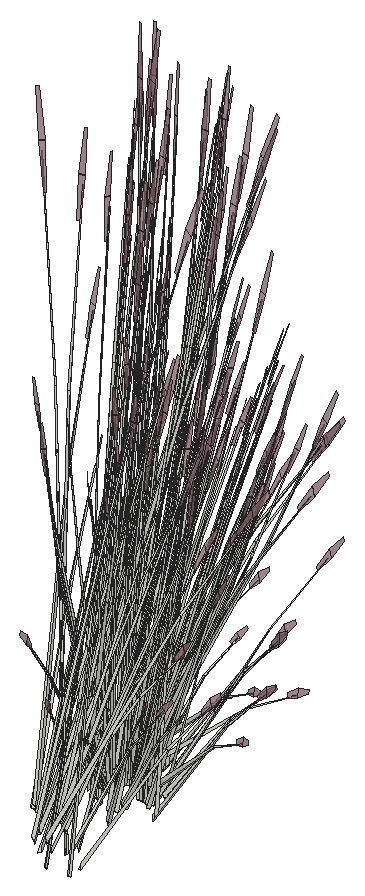
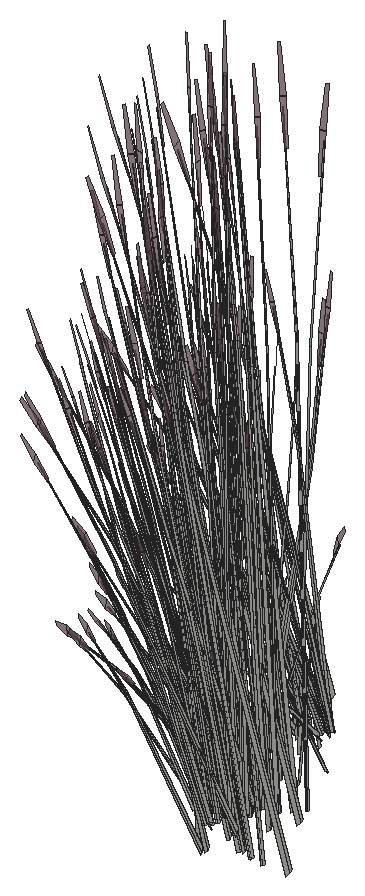
# SketchUp Ruby script. Lengths in inches.
U = 1.inch
M = Sketchup.active_model
def pt(a) = Geom::Point3d.new(a.map { |v| v * U })
def face(e, loops, mat)
  f = e.add_face(loops[0].map { |a| pt(a) })
  loops[1..].each { |l| e.add_face(l.map { |a| pt(a) }).erase! }
  f.material = f.back_material = mat if mat
  f
end
# faces: each face lists its corners as indices into pts; further lists are holes
def faces(e, pts, list, mat = nil) = list.each { |f| face(e, (f[0].is_a?(Array) ? f : [f]).map { |l| l.map { |i| pts[i] } }, mat) }
# xy, xz, yz: faces in a plane at the given z, y or x. An outline is a flat list of corners, or four numbers for a rectangle; further outlines are holes
def ring(l) = l.size == 4 ? [[l[0], l[1]], [l[2], l[1]], [l[2], l[3]], [l[0], l[3]]] : l.each_slice(2).to_a
def flat(e, list, mat, &to3) = list.each { |f| face(e, (f[0].is_a?(Array) ? f : [f]).map { |l| ring(l).map { |u, v| to3.(u, v) } }, mat) }
def xy(e, z, list, mat = nil) = flat(e, list, mat) { |x, y| [x, y, z] }
def xz(e, y, list, mat = nil) = flat(e, list, mat) { |x, z| [x, y, z] }
def yz(e, x, list, mat = nil) = flat(e, list, mat) { |y, z| [x, y, z] }
def lines(e, pts, list) = list.each { |a, b| e.add_line(pt(pts[a]), pt(pts[b])) }
# prism: a flat outline (further loops are holes) pulled along v
def prism(e, loops, v, mat = nil)
  f = face(e, loops, mat); d = Geom::Vector3d.new(v.map { |x| x * U })
  f.pushpull(f.normal.samedirection?(d) ? d.length : -d.length)
end
def box(e, o, s, mat = nil) = prism(e, [[o, [o[0] + s[0], o[1], o[2]], [o[0] + s[0], o[1] + s[1], o[2]], [o[0], o[1] + s[1], o[2]]]], [0, 0, s[2]], mat)
def at(x, y, z, deg = 0) = Geom::Transformation.translation(pt([x, y, z])) * Geom::Transformation.rotation(ORIGIN, Z_AXIS, deg.degrees)
def axes(o, x, y, z) = Geom::Transformation.new([*x, 0, *y, 0, *z, 0, *pt(o).to_a, 1])
def part(name) = M.definitions.add(name)
# library, detail: a bought-in or finely detailed component or shape, given as its bounding box
def library(name, o, s) = part(name).tap { |d| box(d.entities, o, s) }
def detail(e, o, s) = box(e.add_group.entities, o, s)
def put(e, d, t, mat = nil) = e.add_instance(d, t).tap { |i| i.material = mat if mat }
def group(e, t, mat = nil) = e.add_group.tap { |g| g.transformation = t; g.material = mat if mat }.entities
root = M.entities
M.materials.add("LightPink_Translucent").color = [144, 107, 117]
M.materials["LightPink_Translucent"].alpha = 0.75
c1 = part("blade")
p = [[2.15,0.21,22],[0,0.17,0],[0.09,0.45,0],[2.18,0.31,22],[2.29,0.31,22],[0.38,0.45,0],
  [2.48,0.24,33],[2.49,0.24,33],[2.48,0.22,33]]
faces(c1.entities,p,[[0,1,2,3],[4,5,2,3],[6,3,4,7],[8,0,3,6]])
c2 = part("seeds")
p = [[0.3,-0.1,1.38],[-0.01,-0.03,1.59],[-0.01,-0.03,0.03],[0.14,-0.07,-0.07],[0.29,-0.03,3],[0.15,0.01,3.11]]
faces(c2.entities,p,[[0,1,2,3],[1,0,4,5]],"LightPink_Translucent")
c3 = part("blade with seeds")
put(c3.entities,c1,at(0,0,0))
put(c3.entities,c2,axes([2.4,0.25,30.99],[1.5799,-0.05474,1.17369],[-0.12525,1.92788,0.29478],[-0.07173,-0.02425,1.56792]))
put(root,c3,axes([298.54,469.3,2.02],[0,0.65246,-0.49651],[-1.00089,0,0],[0,0.1486,1.57504]))
put(root,c3,axes([296.04,469.375,3.875],[-0.3323,-0.11241,1.71376],[0.68769,-0.4716,0.13857],[0.42861,0.21275,0.73262]))
put(root,c3,axes([295.54,477.44,4.72],[-0.00864,-0.12985,1.74944],[-0.72937,-0.3753,-0.27667],[0.11277,-0.2275,0.14031]))
put(root,c3,axes([296.1,467.9,4.47],[-0.77304,-0.33901,1.38283],[0.81626,-0.52782,0.59665],[0.24941,0.31809,1.33663]))
put(root,c3,axes([293.07,478.08,3.875],[-0.16657,0.22426,1.71376],[-0.69879,-0.4641,0.13857],[0.31524,-0.28926,0.73262]))
put(root,c3,axes([295.34,476.97,4.71],[-0.09085,0.04984,1.77383],[-0.89014,-0.16814,-0.16761],[-0.03222,-0.21748,0.31391]))
put(root,c3,axes([297.27,470.66,2.77],[-0.5037,-0.18761,1.1486],[0.6504,-0.19062,0.84392],[0.17543,0.16147,0.25299]))
put(root,c3,axes([295.5,471.19,5.03],[0.53309,-0.55848,-0.1216],[0.77201,0.32175,-0.67495],[0.26836,0.15779,1.02557]))
put(root,c3,axes([292.62,476.35,2.77],[0.11476,0.38047,1.1486],[-0.63664,-0.21072,0.84392],[0.06851,-0.19481,0.25299]))
put(root,c3,axes([293.97,478.18,4.68],[-0.64041,-0.4384,-0.51099],[0.67652,-0.38394,-0.3958],[0.09744,-0.22274,0.97773]))
put(root,c3,axes([296.52,471.13,2.375],[0.55932,0.6538,0],[-0.93577,0.36461,-0.51607],[-0.21313,0.08304,1.63711]))
put(root,c3,axes([294.8,471.65,4.71],[0.00265,-0.07899,1.77383],[0.76665,-0.34851,-0.16761],[0.2663,0.12439,0.31391]))
put(root,c3,axes([297.41,471.35,1.49],[0.06518,-0.0942,1.76342],[0.82057,-0.27742,-0.26939],[0.24877,0.14358,0.30037]))
put(root,c3,axes([296.33,469.21,2.09],[0.32803,0.59738,-0.69212],[-0.94492,0.21515,-0.18165],[0.03626,0.20229,1.52773]))
put(root,c3,axes([296.13,470.91,4.68],[0.88277,-0.1551,-0.51099],[0.15442,0.58737,-0.3958],[0.23711,0.16832,0.97773]))
put(root,c3,axes([293.68,471,5.05],[0.2697,-0.50175,0.35414],[0.78684,0.14635,-0.4572],[0.07215,0.20201,0.87481]))
put(root,c3,axes([294.65,478.41,5.03],[-0.98321,-0.03233,-0.1216],[0.02687,-0.61208,-0.67495],[0.0683,-0.23574,1.02557]))
put(root,c3,axes([294.58,478.02,4.53],[0.60531,-0.34352,-0.35414],[0.573,0.39225,0.4572],[0.08718,-0.19929,0.87481]))
put(root,c3,axes([297.35,471.51,2.67],[-0.57368,-0.02046,1.0506],[0.37886,-0.43461,0.58006],[0.22663,0.15441,0.8241]))
put(root,c3,axes([295.7,471.39,4.73],[-0.4066,0.41448,0.0643],[-0.57901,-0.24131,0.50621],[0.18719,0.13288,0.77189]))
put(root,c3,axes([294.74,472.79,5.65],[0.61821,-0.37431,-0.06488],[0.56645,0.40995,-0.29416],[0.03988,0.11616,0.97024]))
put(root,c3,axes([295.87,471.28,4.73],[-0.88979,0.14973,0.48003],[-0.15442,-0.58737,0.3958],[0.20926,0.17311,0.9933]))
put(root,c3,axes([295.48,470.46,2.59],[0.01579,-0.21629,1.43002],[0.75442,-0.24159,-0.30754],[0.23289,0.25887,0.61141]))
put(root,c3,axes([295.33,477.8125,1.49],[-0.1339,-0.0514,1.76342],[-0.34394,-0.57425,-0.26939],[0.23202,-0.15583,0.30037]))
put(root,c3,axes([293.44,471.46,4.73],[-0.6592,0.22175,0.0643],[-0.32265,-0.40436,0.50621],[0.06366,0.17825,0.77189]))
put(root,c3,axes([293.42,471.21,5.03],[0.87543,-0.30377,-0.1216],[0.4302,0.53915,-0.67495],[0.1155,0.2272,1.02557]))
put(root,c3,axes([293.67,471.41,5.0625],[-0.88151,-0.17057,0.53283],[0.30143,-0.56078,0.43934],[0.05297,0.22053,1.10256]))
put(root,c3,axes([294.57,478.15,4.73],[0.63704,0.44518,0.48003],[-0.67652,0.38394,0.3958],[0.11751,-0.20886,0.9933]))
put(root,c3,axes([294.81,478.2,4.73],[0.73517,0.0304,0.0643],[-0.02016,0.45906,0.50621],[0.07693,-0.17585,0.77189]))
put(root,c3,axes([293.58,471.33,1.49],[0.14478,-0.0355,1.76342],[0.8709,0.19542,-0.26939],[0.02547,0.22025,0.30037]))
put(root,c3,axes([294.26,478.51,5.05],[-0.60531,0.34352,0.35414],[-0.573,-0.39225,-0.4572],[0.08718,-0.19929,0.87481]))
put(root,c3,axes([295.33,479.43,4.98],[0.4673,-0.51481,-0.71045],[0.81887,0.36587,0.08574],[0.27902,-0.18652,1.00501]))
put(root,c3,axes([290.28,477.93,2.375],[-0.55932,-0.6538,0],[0.93577,-0.36461,-0.51607],[0.21313,-0.08304,1.63711]))
put(root,c3,axes([295.3,479.19,4.68],[-0.22982,-0.59576,-0.51099],[0.87033,-0.10422,-0.3958],[0.24941,-0.16002,0.97773]))
put(root,c3,axes([294.17,471.1875,4.68],[0.87941,0.16356,-0.51099],[-0.30143,0.56078,-0.3958],[0.08064,0.22578,0.97773]))
put(root,c3,axes([294.67,470.03,3.875],[-0.2045,-0.20949,1.71376],[0.94495,-0.17636,0.13857],[0.21357,0.32887,0.73262]))
put(root,c3,axes([295.72,479.62,5.03],[-0.82753,-0.35977,-0.1216],[0.47675,-0.52101,-0.67495],[0.2338,-0.18111,1.02557]))
put(root,c3,axes([293.77,471.53,4.53],[-0.2697,0.50175,-0.35414],[-0.78684,-0.14635,0.4572],[0.07215,0.20201,0.87481]))
put(root,c3,axes([291.04,477.83,2.02],[0.83726,-0.32623,-0.49651],[0.50045,0.58498,0],[0.19069,-0.0743,1.57504]))
put(root,c3,axes([296,478.96,2.59],[-0.31959,-0.01933,1.43002],[-0.32741,-0.51843,-0.30754],[0.39262,-0.14666,0.61141]))
put(root,c3,axes([297.75,479.46,4.71],[-0.11685,-0.00496,1.77383],[-0.48522,-0.53096,-0.16761],[0.19486,-0.17458,0.31391]))
put(root,c3,axes([292.03,479.17,2.06],[0.60257,-0.49041,-0.62353],[0.74854,0.44469,-0.16365],[0.24146,-0.12234,1.37633]))
put(root,c3,axes([296.37,478.01,2.77],[-0.29798,0.33213,1.1486],[-0.25612,-0.44624,0.84392],[0.24611,-0.11182,0.25299]))
put(root,c3,axes([293.85,471.08,4.98],[0.42698,0.53052,-0.71045],[-0.87893,0.29566,0.08574],[0.09984,0.25633,1.00501]))
put(root,c3,axes([295.95,479.25,4.53],[0.77872,-0.09325,-0.35414],[0.20563,0.53305,0.4572],[0.22316,-0.14318,0.87481]))
put(root,c3,axes([293.21,472.42,4.72],[0.1134,0.10507,1.74944],[0.91515,0.04128,-0.27667],[0.09203,0.23172,0.14031]))
put(root,c3,axes([291.375,479.74,2.67],[-0.10425,-0.7445,-0.29095],[1.08575,-0.04502,-0.50002],[0.19119,-0.09917,1.59708]))
put(root,c3,axes([295.3125,479.57,5.05],[-0.77872,0.09325,0.35414],[-0.20563,-0.53305,-0.4572],[0.22316,-0.14318,0.87481]))
put(root,c3,axes([291.23,478.09,2.03],[0.83462,0.16144,-0.30978],[-0.21015,0.56852,0.30978],[0.16826,-0.06556,1.38974]))
put(root,c3,axes([296.02,479.48,4.73],[0.61415,0.2744,0.0643],[-0.35756,0.39076,0.50621],[0.1969,-0.12633,0.77189]))
put(root,c3,axes([295.85,479.37,4.73],[0.22187,0.60049,0.48003],[-0.87033,0.10422,0.3958],[0.25651,-0.14123,0.9933]))
put(root,c3,axes([298.19,480.1,4.72],[0.12414,-0.09938,1.74944],[-0.15889,-0.60963,-0.27667],[0.31148,-0.11559,0.14031]))
put(root,c3,axes([295.75,481.02,5.03],[-0.45012,-0.59081,-0.1216],[0.79888,-0.29033,-0.67495],[0.33665,-0.07795,1.02557]))
put(root,c3,axes([295.71,480.51,4.68],[0.24236,-0.59349,-0.51099],[0.83094,0.20343,-0.3958],[0.33455,-0.05442,0.97773]))
put(root,c3,axes([294.4,478.1,2.375],[0.55932,-0.6538,0],[0.93577,0.36461,-0.51607],[0.21313,0.08304,1.63711]))
put(root,c3,axes([296.6,480.68,1.98],[-0.57619,0.0783,1.41583],[-0.09171,-0.62326,0.08104],[0.40356,-0.09434,0.80566]))
put(root,c3,axes([297.65,480.13,2.26],[-0.55463,-0.41721,-0.06488],[0.60744,-0.38228,-0.29416],[0.17212,-0.02691,0.97024]))
put(root,c3,axes([293.91,478.4375,2.48],[-0.83726,-0.32623,0.49651],[0.50045,-0.58498,0],[0.19069,0.0743,1.57504]))
put(root,c3,axes([295.55,480.73,4.98],[0.78611,-0.28816,-0.71045],[0.4381,0.59317,0.08574],[0.37982,-0.06738,1.00501]))
put(root,c3,axes([291.55,483.7,4.72],[-0.00864,-0.12985,1.74944],[-0.72937,-0.3753,-0.27667],[0.11277,-0.2275,0.14031]))
put(root,c3,axes([289.08,484.34,3.875],[-0.16657,0.22426,1.71376],[-0.69879,-0.4641,0.13857],[0.31524,-0.28926,0.73262]))
put(root,c3,axes([292.03,479.71,2.36],[-0.74176,0.59212,0.45755],[-0.88124,-0.52269,0.17955],[0.17882,-0.05909,1.58856]))
put(root,c3,axes([295.44,480.84,5.05],[-0.74348,-0.18202,0.35414],[0.21685,-0.53102,-0.4572],[0.29933,-0.04869,0.87481]))
put(root,c3,axes([290.35,479.26,1.59],[-0.88056,0.26122,1.28929],[-0.28027,-0.74951,0.50096],[0.54072,0.01247,1.46642]))
put(root,c3,axes([292.71,479.45,2.62],[0.17258,-0.58229,0.1448],[0.84319,0.10108,-0.41347],[0.15345,0.05979,1.26744]))
put(root,c3,axes([297.23,480.27,1.49],[-0.04675,-0.09906,1.76342],[0.32428,-0.57943,-0.26939],[0.32711,-0.00833,0.30037]))
put(root,c3,axes([292.35,479.61,2.72],[-0.53742,-0.54764,0.44739],[0.81403,-0.38564,-0.21531],[0.17391,0.06776,1.43643]))
put(root,c3,axes([292.63,479.64,2.67],[0.90324,-0.43318,-0.29095],[0.60064,0.61207,-0.50002],[0.22285,0.06216,1.59708]))
put(root,c3,axes([296.22,480.79,4.53],[0.74348,0.18202,-0.35414],[-0.21685,0.53102,0.4572],[0.29933,-0.04869,0.87481]))
put(root,c3,axes([294.9,478.49,2.02],[0.83726,0.32623,-0.49651],[-0.50045,0.58498,0],[0.19069,0.0743,1.57504]))
put(root,c3,axes([293.32,480.35,2.21],[1.00089,0,0],[0,0.67548,0],[0,0,1.78407]))
put(root,c3,axes([293.6,478.77,2.47],[-0.96132,0.17317,0.17642],[-0.23737,-0.64447,0.35086],[0.08574,0.0939,1.60407]))
put(root,c3,axes([294.19,480.13,3.875],[-0.37107,0.01478,1.71376],[0.24616,-0.64047,0.13857],[0.5288,0.03961,0.73262]))
put(root,c3,axes([294.67,478.73,2.03],[0.21015,0.56852,-0.30978],[-0.83462,0.16144,0.30978],[0.16826,0.06556,1.38974]))
put(root,c3,axes([296.11,481.01,4.73],[0.32857,0.44488,0.0643],[-0.59916,0.21775,0.50621],[0.26412,-0.04296,0.77189]))
put(root,c3,axes([292.99,480.01,2.38],[-1.13071,-0.13747,0.49198],[0.23011,-0.77639,0.19306],[0.16524,0.07497,1.70813]))
put(root,c3,axes([296.05,480.85,4.73],[-0.25275,0.59491,0.48003],[-0.83094,-0.20343,0.3958],[0.32677,-0.03575,0.9933]))
put(root,c3,axes([291.35,484.07,1.49],[-0.1339,-0.0514,1.76342],[-0.34394,-0.57425,-0.26939],[0.23202,-0.15583,0.30037]))
put(root,c3,axes([293.18,481.85,2.18],[0.93921,-0.22138,-0.19198],[0.33003,0.6377,0.00008],[0.10367,-0.02447,1.73897]))
put(root,c3,axes([293.29,480.64,2.21],[0.62448,0.42144,0],[-0.62448,0.42144,0],[0,0,1.69266]))
put(root,c3,axes([290.59,484.41,4.73],[0.63704,0.44518,0.48003],[-0.67652,0.38394,0.3958],[0.11751,-0.20886,0.9933]))
put(root,c3,axes([290.82,484.46,4.73],[0.73517,0.0304,0.0643],[-0.02016,0.45906,0.50621],[0.07693,-0.17585,0.77189]))
put(root,c3,axes([293.68,479.74,2.06],[0.9306,0.10697,-0.62353],[-0.19638,0.65984,-0.16365],[0.27771,0.07995,1.37633]))
put(root,c3,axes([297.8,480.89,2.77],[-0.55274,0.10771,1.1486],[0.26018,-0.44517,0.84392],[0.29323,0.03046,0.25299]))
put(root,c3,axes([291.34,485.69,4.98],[0.4673,-0.51481,-0.71045],[0.81887,0.36587,0.08574],[0.27902,-0.18652,1.00501]))
put(root,c3,axes([291.32,485.45,4.68],[-0.22982,-0.59576,-0.51099],[0.87033,-0.10422,-0.3958],[0.24941,-0.16002,0.97773]))
put(root,c3,axes([293.29,480.15,2.72],[0.43405,-0.58792,0.44739],[0.90188,0.28295,-0.21531],[0,0.13553,1.43643]))
put(root,c3,axes([297.54,482.78,4.71],[-0.08089,-0.05712,1.77383],[0.17695,-0.61228,-0.16761],[0.31864,-0.03912,0.31391]))
put(root,c3,axes([291.73,485.88,5.03],[-0.82753,-0.35977,-0.1216],[0.47675,-0.52101,-0.67495],[0.2338,-0.18111,1.02557]))
put(root,c3,axes([293.2,479.95,2.21],[0.53742,0.54764,-0.44739],[-0.81403,0.38564,0.21531],[0.17391,0.06776,1.43643]))
put(root,c3,axes([296.84,482.27,3.93],[-0.17122,-0.54847,-0.03492],[0.80929,-0.12609,-0.15832],[0.169,0.03477,0.52218]))
put(root,c3,axes([294.74,482.25,5.03],[0.0479,-0.66354,-0.1216],[0.90696,0.01814,-0.67495],[0.3493,0.04609,1.02557]))
put(root,c3,axes([295.5625,480.48,2.48],[0,-0.65246,0.49651],[1.00089,0,0],[0,0.1486,1.57504]))
put(root,c3,axes([293.66,480.28,2.62],[0.83351,-0.19028,0.1448],[0.29189,0.54335,-0.41347],[0,0.11958,1.26744]))
put(root,c3,axes([294.6,481.99,5.05],[-0.50902,-0.40851,0.35414],[0.58122,-0.38671,-0.4572],[0.29531,0.05884,0.87481]))
put(root,c3,axes([292.02,485.22,2.59],[-0.31959,-0.01933,1.43002],[-0.32741,-0.51843,-0.30754],[0.39262,-0.14666,0.61141]))
put(root,c3,axes([293.77,485.72,4.71],[-0.11685,-0.00496,1.77383],[-0.48522,-0.53096,-0.16761],[0.19486,-0.17458,0.31391]))
put(root,c3,axes([296.76,481.61,2.59],[-0.21545,-0.16047,1.43002],[0.28033,-0.53085,-0.30754],[0.43591,0.07191,0.61141]))
put(root,c3,axes([288.04,485.43,2.06],[0.60257,-0.49041,-0.62353],[0.74854,0.44469,-0.16365],[0.24146,-0.12234,1.37633]))
put(root,c3,axes([292.39,484.27,2.77],[-0.29798,0.33213,1.1486],[-0.25612,-0.44624,0.84392],[0.24611,-0.11182,0.25299]))
put(root,c3,axes([292.91,482.19,2.2],[0.90188,0.29293,0],[-0.43405,0.60866,0],[0,0,1.74954]))
put(root,c3,axes([291.96,485.51,4.53],[0.77872,-0.09325,-0.35414],[0.20563,0.53305,0.4572],[0.22316,-0.14318,0.87481]))
put(root,c3,axes([295.53,481.85,4.72],[0.19191,-0.01103,1.74944],[0.52639,-0.5069,-0.27667],[0.34136,0.06691,0.14031]))
put(root,c3,axes([291.33,485.83,5.05],[-0.77872,0.09325,0.35414],[-0.20563,-0.53305,-0.4572],[0.22316,-0.14318,0.87481]))
put(root,c3,axes([294.78,481.93,4.98],[0.89428,0.01571,-0.71045],[-0.06006,0.66153,0.08574],[0.37886,0.06981,1.00501]))
put(root,c3,axes([296.24,480.59,2.375],[1.11865,0,0],[0,0.72922,-0.51607],[0,0.16609,1.63711]))
put(root,c3,axes([295.8,480.96,2.2],[-1.1181,-0.00522,-0.04976],[0,-0.72922,0.49943],[-0.03514,0.166,1.58352]))
put(root,c3,axes([293.375,480.33,2.67],[1.00749,0.31132,-0.29095],[-0.48511,0.65709,-0.50002],[0.03166,0.16133,1.59708]))
put(root,c3,axes([292.03,485.75,4.73],[0.61415,0.2744,0.0643],[-0.35756,0.39076,0.50621],[0.1969,-0.12633,0.77189]))
put(root,c3,axes([295.32,482.2,4.53],[0.50902,0.40851,-0.35414],[-0.58122,0.38671,0.4572],[0.29531,0.05884,0.87481]))
put(root,c3,axes([295.5625,481.07,2.03],[-0.62448,0.40708,-0.30978],[-0.62448,-0.40708,0.30978],[0,0.13112,1.38974]))
put(root,c3,axes([291.86,485.63,4.73],[0.22187,0.60049,0.48003],[-0.87033,0.10422,0.3958],[0.25651,-0.14123,0.9933]))
put(root,c3,axes([294.21,486.36,4.72],[0.12414,-0.09938,1.74944],[-0.15889,-0.60963,-0.27667],[0.31148,-0.11559,0.14031]))
put(root,c3,axes([295.06,482.36,4.73],[-0.04505,0.49615,0.0643],[-0.68022,-0.0136,0.50621],[0.26056,0.05192,0.77189]))
put(root,c3,axes([295.12,482.2,4.73],[-0.65964,0.42992,0.48003],[-0.5689,-0.45657,0.3958],[0.30948,0.0793,0.9933]))
put(root,c3,axes([293.02,482.7,5.05],[-0.13817,-0.52554,0.35414],[0.78985,-0.13877,-0.4572],[0.21215,0.1506,0.87481]))
put(root,c3,axes([295.99,481.08,2.02],[0,0.65246,-0.49651],[-1.00089,0,0],[0,0.1486,1.57504]))
put(root,c3,axes([293.49,481.16,3.875],[-0.3323,-0.11241,1.71376],[0.68769,-0.4716,0.13857],[0.42861,0.21275,0.73262]))
put(root,c3,axes([293.56,479.68,4.47],[-0.77304,-0.33901,1.38283],[0.81626,-0.52782,0.59665],[0.24941,0.31809,1.33663]))
put(root,c3,axes([291.76,487.28,5.03],[-0.45012,-0.59081,-0.1216],[0.79888,-0.29033,-0.67495],[0.33665,-0.07795,1.02557]))
put(root,c3,axes([291.72,486.77,4.68],[0.24236,-0.59349,-0.51099],[0.83094,0.20343,-0.3958],[0.33455,-0.05442,0.97773]))
put(root,c3,axes([290.41,484.36,2.375],[0.55932,-0.6538,0],[0.93577,0.36461,-0.51607],[0.21313,0.08304,1.63711]))
put(root,c3,axes([294.72,482.4375,2.77],[-0.5037,-0.18761,1.1486],[0.6504,-0.19062,0.84392],[0.17543,0.16147,0.25299]))
put(root,c3,axes([292.95,482.97,5.03],[0.53309,-0.55848,-0.1216],[0.77201,0.32175,-0.67495],[0.26836,0.15779,1.02557]))
put(root,c3,axes([292.61,486.94,1.98],[-0.57619,0.0783,1.41583],[-0.09171,-0.62326,0.08104],[0.40356,-0.09434,0.80566]))
put(root,c3,axes([293.66,486.39,2.26],[-0.55463,-0.41721,-0.06488],[0.60744,-0.38228,-0.29416],[0.17212,-0.02691,0.97024]))
put(root,c3,axes([291.57,486.99,4.98],[0.78611,-0.28816,-0.71045],[0.4381,0.59317,0.08574],[0.37982,-0.06738,1.00501]))
put(root,c3,axes([292.25,483.43,4.71],[0.00265,-0.07899,1.77383],[0.76665,-0.34851,-0.16761],[0.2663,0.12439,0.31391]))
put(root,c3,axes([294.86,483.13,1.49],[0.06518,-0.0942,1.76342],[0.82057,-0.27742,-0.26939],[0.24877,0.14358,0.30037]))
put(root,c3,axes([293.78,480.99,2.09],[0.32803,0.59738,-0.69212],[-0.94492,0.21515,-0.18165],[0.03626,0.20229,1.52773]))
put(root,c3,axes([293.58,482.69,4.68],[0.88277,-0.1551,-0.51099],[0.15442,0.58737,-0.3958],[0.23711,0.16832,0.97773]))
put(root,c3,axes([291.45,487.1,5.05],[-0.74348,-0.18202,0.35414],[0.21685,-0.53102,-0.4572],[0.29933,-0.04869,0.87481]))
put(root,c3,axes([286.36,485.52,1.59],[-0.88056,0.26122,1.28929],[-0.28027,-0.74951,0.50096],[0.54072,0.01247,1.46642]))
put(root,c3,axes([294.8,483.29,2.67],[-0.57368,-0.02046,1.0506],[0.37886,-0.43461,0.58006],[0.22663,0.15441,0.8241]))
put(root,c3,axes([293.24,486.53,1.49],[-0.04675,-0.09906,1.76342],[0.32428,-0.57943,-0.26939],[0.32711,-0.00833,0.30037]))
put(root,c3,axes([293.15,483.18,4.73],[-0.4066,0.41448,0.0643],[-0.57901,-0.24131,0.50621],[0.18719,0.13288,0.77189]))
put(root,c3,axes([292.19,484.57,5.65],[0.61821,-0.37431,-0.06488],[0.56645,0.40995,-0.29416],[0.03988,0.11616,0.97024]))
put(root,c3,axes([293.32,483.06,4.73],[-0.88979,0.14973,0.48003],[-0.15442,-0.58737,0.3958],[0.20926,0.17311,0.9933]))
put(root,c3,axes([288.64,485.9,2.67],[0.90324,-0.43318,-0.29095],[0.60064,0.61207,-0.50002],[0.22285,0.06216,1.59708]))
put(root,c3,axes([292.23,487.05,4.53],[0.74348,0.18202,-0.35414],[-0.21685,0.53102,0.4572],[0.29933,-0.04869,0.87481]))
put(root,c3,axes([292.93,482.24,2.59],[0.01579,-0.21629,1.43002],[0.75442,-0.24159,-0.30754],[0.23289,0.25887,0.61141]))
put(root,c3,axes([290.92,484.75,2.02],[0.83726,0.32623,-0.49651],[-0.50045,0.58498,0],[0.19069,0.0743,1.57504]))
put(root,c3,axes([290.87,482.99,5.03],[0.87543,-0.30377,-0.1216],[0.4302,0.53915,-0.67495],[0.1155,0.2272,1.02557]))
put(root,c3,axes([290.21,486.39,3.875],[-0.37107,0.01478,1.71376],[0.24616,-0.64047,0.13857],[0.5288,0.03961,0.73262]))
put(root,c3,axes([290.6875,485,2.03],[0.21015,0.56852,-0.30978],[-0.83462,0.16144,0.30978],[0.16826,0.06556,1.38974]))
